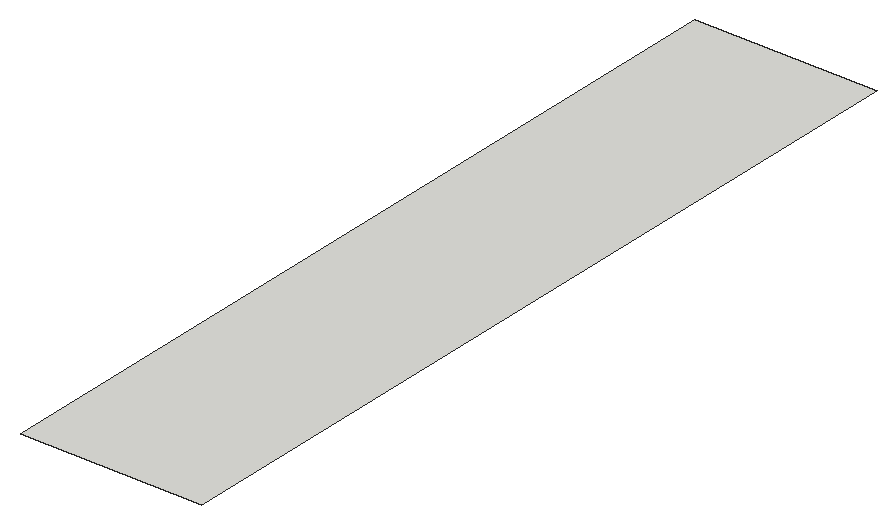
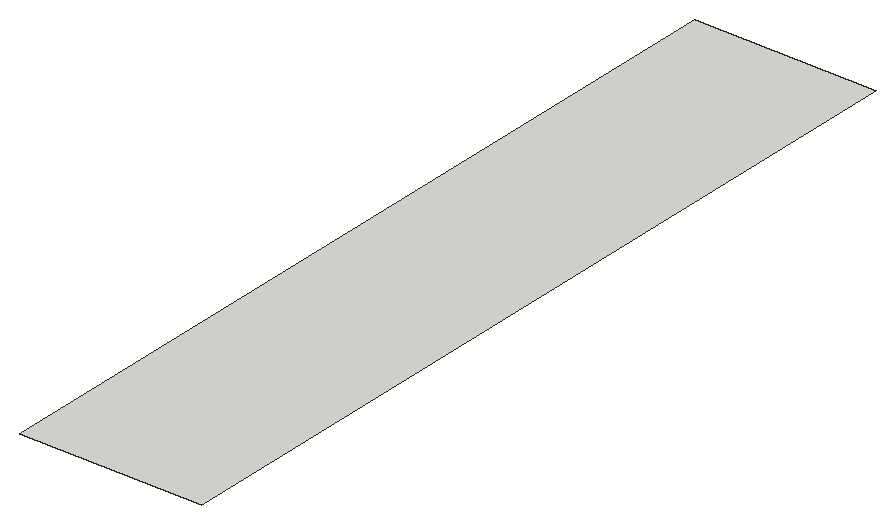
# SketchUp Ruby script. Lengths in inches.
U = 1.inch
M = Sketchup.active_model
def pt(a) = Geom::Point3d.new(a.map { |v| v * U })
def face(e, loops, mat)
  f = e.add_face(loops[0].map { |a| pt(a) })
  loops[1..].each { |l| e.add_face(l.map { |a| pt(a) }).erase! }
  f.material = f.back_material = mat if mat
  f
end
# faces: each face lists its corners as indices into pts; further lists are holes
def faces(e, pts, list, mat = nil) = list.each { |f| face(e, (f[0].is_a?(Array) ? f : [f]).map { |l| l.map { |i| pts[i] } }, mat) }
# xy, xz, yz: faces in a plane at the given z, y or x. An outline is a flat list of corners, or four numbers for a rectangle; further outlines are holes
def ring(l) = l.size == 4 ? [[l[0], l[1]], [l[2], l[1]], [l[2], l[3]], [l[0], l[3]]] : l.each_slice(2).to_a
def flat(e, list, mat, &to3) = list.each { |f| face(e, (f[0].is_a?(Array) ? f : [f]).map { |l| ring(l).map { |u, v| to3.(u, v) } }, mat) }
def xy(e, z, list, mat = nil) = flat(e, list, mat) { |x, y| [x, y, z] }
def xz(e, y, list, mat = nil) = flat(e, list, mat) { |x, z| [x, y, z] }
def yz(e, x, list, mat = nil) = flat(e, list, mat) { |y, z| [x, y, z] }
def lines(e, pts, list) = list.each { |a, b| e.add_line(pt(pts[a]), pt(pts[b])) }
# prism: a flat outline (further loops are holes) pulled along v
def prism(e, loops, v, mat = nil)
  f = face(e, loops, mat); d = Geom::Vector3d.new(v.map { |x| x * U })
  f.pushpull(f.normal.samedirection?(d) ? d.length : -d.length)
end
def box(e, o, s, mat = nil) = prism(e, [[o, [o[0] + s[0], o[1], o[2]], [o[0] + s[0], o[1] + s[1], o[2]], [o[0], o[1] + s[1], o[2]]]], [0, 0, s[2]], mat)
def at(x, y, z, deg = 0) = Geom::Transformation.translation(pt([x, y, z])) * Geom::Transformation.rotation(ORIGIN, Z_AXIS, deg.degrees)
def axes(o, x, y, z) = Geom::Transformation.new([*x, 0, *y, 0, *z, 0, *pt(o).to_a, 1])
def part(name) = M.definitions.add(name)
# library, detail: a bought-in or finely detailed component or shape, given as its bounding box
def library(name, o, s) = part(name).tap { |d| box(d.entities, o, s) }
def detail(e, o, s) = box(e.add_group.entities, o, s)
def put(e, d, t, mat = nil) = e.add_instance(d, t).tap { |i| i.material = mat if mat }
def group(e, t, mat = nil) = e.add_group.tap { |g| g.transformation = t; g.material = mat if mat }.entities
root = M.entities
xy(root,92.87,[[277.93,203.17,281.86,221.48]])
